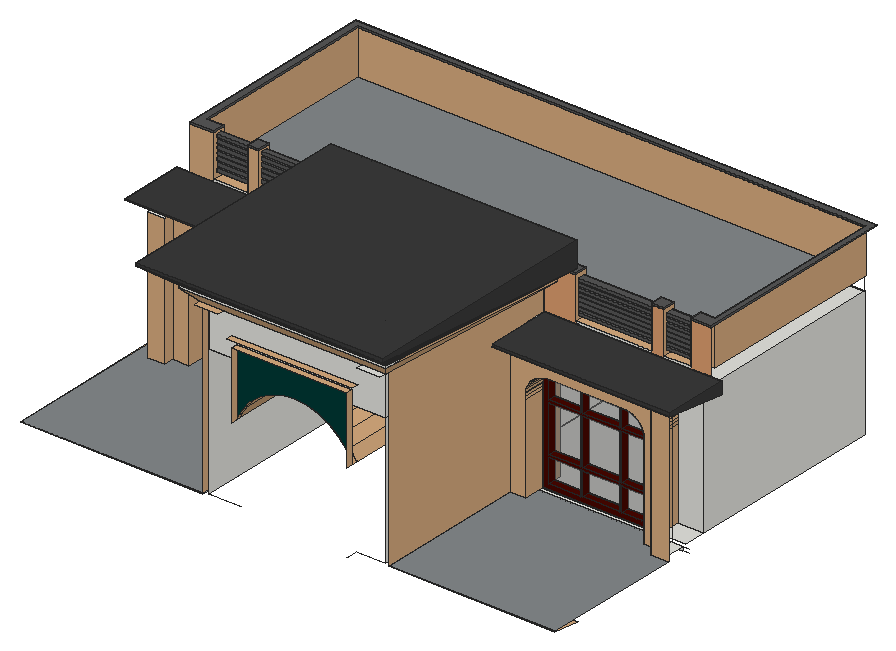
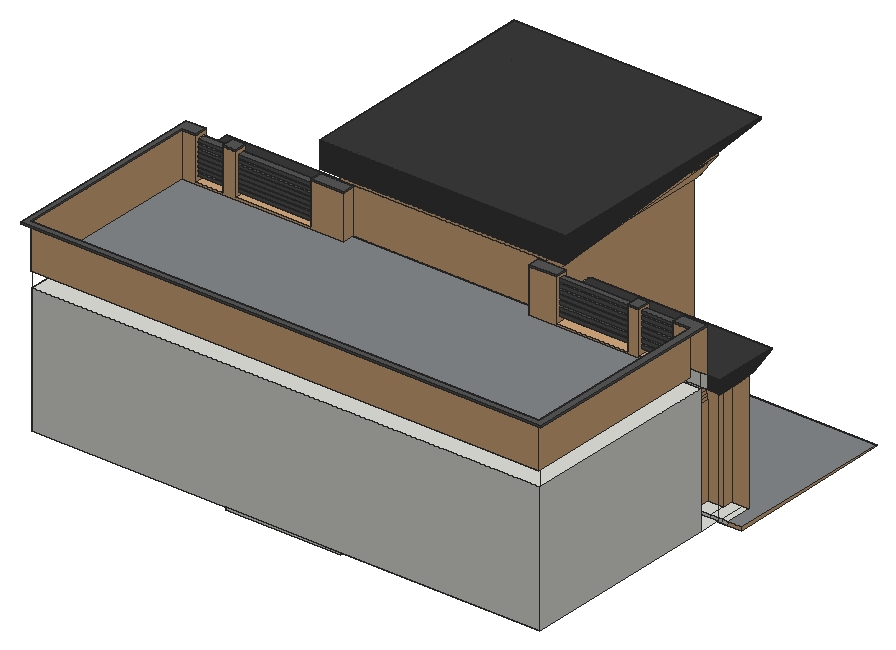
# SketchUp Ruby script. Lengths in inches.
U = 1.inch
M = Sketchup.active_model
def pt(a) = Geom::Point3d.new(a.map { |v| v * U })
def face(e, loops, mat)
  f = e.add_face(loops[0].map { |a| pt(a) })
  loops[1..].each { |l| e.add_face(l.map { |a| pt(a) }).erase! }
  f.material = f.back_material = mat if mat
  f
end
# faces: each face lists its corners as indices into pts; further lists are holes
def faces(e, pts, list, mat = nil) = list.each { |f| face(e, (f[0].is_a?(Array) ? f : [f]).map { |l| l.map { |i| pts[i] } }, mat) }
# xy, xz, yz: faces in a plane at the given z, y or x. An outline is a flat list of corners, or four numbers for a rectangle; further outlines are holes
def ring(l) = l.size == 4 ? [[l[0], l[1]], [l[2], l[1]], [l[2], l[3]], [l[0], l[3]]] : l.each_slice(2).to_a
def flat(e, list, mat, &to3) = list.each { |f| face(e, (f[0].is_a?(Array) ? f : [f]).map { |l| ring(l).map { |u, v| to3.(u, v) } }, mat) }
def xy(e, z, list, mat = nil) = flat(e, list, mat) { |x, y| [x, y, z] }
def xz(e, y, list, mat = nil) = flat(e, list, mat) { |x, z| [x, y, z] }
def yz(e, x, list, mat = nil) = flat(e, list, mat) { |y, z| [x, y, z] }
def lines(e, pts, list) = list.each { |a, b| e.add_line(pt(pts[a]), pt(pts[b])) }
# prism: a flat outline (further loops are holes) pulled along v
def prism(e, loops, v, mat = nil)
  f = face(e, loops, mat); d = Geom::Vector3d.new(v.map { |x| x * U })
  f.pushpull(f.normal.samedirection?(d) ? d.length : -d.length)
end
def box(e, o, s, mat = nil) = prism(e, [[o, [o[0] + s[0], o[1], o[2]], [o[0] + s[0], o[1] + s[1], o[2]], [o[0], o[1] + s[1], o[2]]]], [0, 0, s[2]], mat)
def at(x, y, z, deg = 0) = Geom::Transformation.translation(pt([x, y, z])) * Geom::Transformation.rotation(ORIGIN, Z_AXIS, deg.degrees)
def axes(o, x, y, z) = Geom::Transformation.new([*x, 0, *y, 0, *z, 0, *pt(o).to_a, 1])
def part(name) = M.definitions.add(name)
# library, detail: a bought-in or finely detailed component or shape, given as its bounding box
def library(name, o, s) = part(name).tap { |d| box(d.entities, o, s) }
def detail(e, o, s) = box(e.add_group.entities, o, s)
def put(e, d, t, mat = nil) = e.add_instance(d, t).tap { |i| i.material = mat if mat }
def group(e, t, mat = nil) = e.add_group.tap { |g| g.transformation = t; g.material = mat if mat }.entities
root = M.entities
M.materials.add("[Blacktop Old 01]").color = [132, 136, 139]
M.materials.add("[Checker Plate]").color = [0, 56, 52]
M.materials.add("[Color C04]").color = [215, 171, 127]
M.materials.add("[Color C04]1").color = [220, 158, 110]
M.materials.add("[Color C08]").color = [71, 7, 0]
M.materials.add("[Color M06]").color = [86, 86, 86]
M.materials.add("[Color M07]").color = [58, 58, 58]
M.materials.add("[Translucent Glass Gray]").color = [128, 128, 128]
M.materials["[Translucent Glass Gray]"].alpha = 0.5
c1 = part("Group\#1")
xy(c1.entities,0,[[0,0,133.1875,11.375]],"[Color C08]")
xy(c1.entities,6.44,[[6.44,0,42.59,11.375],[44.75,0,86.9,11.375],[89.0625,0,126.75,11.375]],"[Color C08]")
xy(c1.entities,37.85,[[6.44,0,42.59,11.375],[44.75,0,86.9,11.375],[89.0625,0,126.75,11.375]],"[Color C08]")
xy(c1.entities,40.75,[[6.44,0,42.59,11.375],[44.75,0,86.9,11.375],[89.0625,0,126.75,11.375]],"[Color C08]")
xy(c1.entities,101.6,[[6.44,0,42.59,11.375],[44.75,0,86.9,11.375],[89.0625,0,126.75,11.375]],"[Color C08]")
xy(c1.entities,104.5,[[6.44,0,42.59,11.375],[44.75,0,86.9,11.375],[89.0625,0,126.75,11.375]],"[Color C08]")
xy(c1.entities,140.62,[[24.51,0,42.59,11.375],[44.75,0,86.9,11.375],[89.0625,0,107.9,11.375]],"[Color C08]")
xy(c1.entities,147.0625,[[0,0,133.1875,11.375]],"[Color C08]")
xz(c1.entities,0,[[[0,0,133.1875,147.0625],[44.75,40.75,86.9,101.6],[89.0625,40.75,126.75,101.6],[6.44,40.75,42.59,101.6],[44.75,104.5,86.9,140.62],[44.75,6.44,86.9,37.85],[89.0625,104.5,89.0625,140.62,107.9,140.62,110.36,140.46,112.78,139.98,115.11,139.1875,117.33,138.1,119.375,136.73,121.23,135.1,122.85,133.25,124.22,131.2,125.3125,128.99,126.1,126.66,126.58,124.24,126.75,121.78,126.75,104.5],[6.44,104.5,6.44,127.03,6.65,127.83,7.8,130.52,9.36,133,11.29,135.21,13.53,137.09,16.03,138.61,18.75,139.72,21.59,140.39,24.51,140.62,42.59,140.62,42.59,104.5],[89.0625,6.44,126.75,37.85],[6.44,6.44,42.59,37.85]]],"[Color C08]")
xz(c1.entities,11.375,[[[0,0,133.1875,147.0625],[44.75,40.75,86.9,101.6],[89.0625,40.75,126.75,101.6],[6.44,40.75,42.59,101.6],[44.75,104.5,86.9,140.62],[44.75,6.44,86.9,37.85],[89.0625,104.5,126.75,104.5,126.75,121.78,126.58,124.24,126.1,126.66,125.3125,128.99,124.22,131.2,122.85,133.25,121.23,135.1,119.375,136.73,117.33,138.1,115.11,139.1875,112.78,139.98,110.36,140.46,107.9,140.62,89.0625,140.62],[6.44,104.5,42.59,104.5,42.59,140.62,24.51,140.62,21.59,140.39,18.75,139.72,16.03,138.61,13.53,137.09,11.29,135.21,9.36,133,7.8,130.52,6.65,127.83,6.44,127.03],[89.0625,6.44,126.75,37.85],[6.44,6.44,42.59,37.85]]],"[Color C08]")
xz(c1.entities,11.375,[[6.44,6.44,42.59,37.85],[44.75,6.44,86.9,37.85],[89.0625,6.44,126.75,37.85],[6.44,40.75,42.59,101.6],[44.75,40.75,86.9,101.6],
  [89.0625,40.75,126.75,101.6],[6.44,104.5,42.59,104.5,42.59,140.62,24.51,140.62,21.59,140.39,18.75,139.72,16.03,138.61,13.53,137.09,11.29,135.21,9.36,133,7.8,130.52,6.65,127.83,6.44,127.03],[44.75,104.5,86.9,140.62],[89.0625,104.5,126.75,104.5,126.75,121.78,126.58,124.24,126.1,126.66,125.3125,128.99,124.22,131.2,122.85,133.25,121.23,135.1,119.375,136.73,117.33,138.1,115.11,139.1875,112.78,139.98,110.36,140.46,107.9,140.62,89.0625,140.62]],"[Translucent Glass Gray]")
yz(c1.entities,0,[[0,0,11.375,147.0625]],"[Color C08]")
yz(c1.entities,6.44,[[0,6.44,11.375,37.85],[0,40.75,11.375,101.6],[0,104.5,11.375,127.03]],"[Color C08]")
yz(c1.entities,42.59,[[0,6.44,11.375,37.85],[0,40.75,11.375,101.6],[0,104.5,11.375,140.62]],"[Color C08]")
yz(c1.entities,44.75,[[0,6.44,11.375,37.85],[0,40.75,11.375,101.6],[0,104.5,11.375,140.62]],"[Color C08]")
yz(c1.entities,86.9,[[0,6.44,11.375,37.85],[0,40.75,11.375,101.6],[0,104.5,11.375,140.62]],"[Color C08]")
yz(c1.entities,89.0625,[[0,6.44,11.375,37.85],[0,40.75,11.375,101.6],[0,104.5,11.375,140.62]],"[Color C08]")
yz(c1.entities,126.75,[[0,6.44,11.375,37.85],[0,40.75,11.375,101.6],[0,104.5,11.375,121.78]],"[Color C08]")
yz(c1.entities,133.1875,[[0,0,11.375,147.0625]],"[Color C08]")
p = [[126.58,11.375,124.24],[126.75,11.375,121.78],[126.75,0,121.78],[126.58,0,124.24],[126.1,11.375,126.66],[126.1,0,126.66],
  [125.3125,11.375,128.99],[125.3125,0,128.99],[6.44,11.375,127.03],[6.65,11.375,127.83],[6.65,0,127.83],[6.44,0,127.03],
  [7.8,11.375,130.52],[7.8,0,130.52],[124.22,11.375,131.2],[124.22,0,131.2],[9.36,11.375,133],[9.36,0,133],
  [122.85,11.375,133.25],[122.85,0,133.25],[11.29,11.375,135.21],[11.29,0,135.21],[121.23,11.375,135.1],[121.23,0,135.1],
  [119.375,11.375,136.73],[119.375,0,136.73],[13.53,11.375,137.09],[13.53,0,137.09],[117.33,11.375,138.1],[117.33,0,138.1],
  [16.03,11.375,138.61],[16.03,0,138.61],[115.11,11.375,139.1875],[115.11,0,139.1875],[18.75,11.375,139.72],[18.75,0,139.72],
  [112.78,11.375,139.98],[112.78,0,139.98],[21.59,11.375,140.39],[21.59,0,140.39],[110.36,11.375,140.46],[110.36,0,140.46],
  [24.51,11.375,140.62],[24.51,0,140.62],[107.9,11.375,140.62],[107.9,0,140.62]]
faces(c1.entities,p,[[0,1,2,3],[4,0,3,5],[6,4,5,7],[8,9,10,11],[9,12,13,10],[14,6,7,15],[12,16,17,13],[18,14,15,19],
  [16,20,21,17],[22,18,19,23],[24,22,23,25],[20,26,27,21],[28,24,25,29],[26,30,31,27],[32,28,29,33],[30,34,35,31],
  [36,32,33,37],[34,38,39,35],[40,36,37,41],[38,42,43,39],[44,40,41,45]],"[Color C08]")
xy(root,271.1875,[[19.375,626.0625,252.9375,820.1875]])
xy(root,273.1875,[[303.29,826.22,323.73,826.22,323.73,826.24],[303.29,826.22,323.73,826.24,323.73,1134.4375,303.29,1134.4375],[323.73,826.24,323.73,1134.4375,462.79,1134.4375,462.79,826.34]])
xy(root,276.1875,[[19.375,784.25,28.375,820.1875],[28.375,784.25,42.875,820.1875],[715.65,784.25,730.375,820.1875],[42.875,798.1875,65.86,820.1875],[228.61,798.1875,252.9375,820.1875],
  [509.3125,798.1875,526.3125,820.1875],[526.3125,798.1875,531.01,820.1875],[694.01,798.1875,715.65,820.1875],[65.86,820.1875,228.61,826.1875],[531.01,820.1875,694.01,826.1875],
  [28.375,826.1875,65.86,857.1875],[65.86,826.1875,228.61,826.1875,228.61,857.1875,258.9375,857.1875,258.9375,826.1875,303.29,826.22,303.29,1134.4375,28.375,1134.4375,28.375,857.1875,65.86,857.1875],[228.61,826.1875,258.9375,857.1875],[509.3125,826.1875,509.3125,857.1875,531.01,857.1875,531.01,826.1875,694.01,826.1875,694.01,857.1875,730.375,857.1875,730.375,1134.4375,462.79,1134.4375,462.79,826.34,503.3125,826.375],[509.3125,826.1875,531.01,857.1875],
  [694.01,826.1875,730.375,857.1875],[303.29,826.22,462.79,826.34,462.79,1134.4375,303.29,1134.4375],[303.29,826.22,462.79,826.34,462.79,826.22]])
xy(root,276.1875,[[0,588.625,252.9375,588.625,252.9375,798.1875,228.61,798.1875,228.61,820.1875,65.86,820.1875,65.86,798.1875,42.875,798.1875,42.875,784.25,19.375,784.25,19.375,820.1875,0,820.1875],[509.3125,588.625,739.375,588.625,739.375,784.25,715.65,784.25,715.65,798.1875,694.01,798.1875,694.01,820.1875,531.01,820.1875,531.01,798.1875,509.3125,798.1875]],"[Blacktop Old 01]")
xy(root,428.8125,[[94.08,798.1875,199.86,857.1875]],"[Color C04]")
xy(root,434.0625,[[561.99,798.1875,665.6,857.1875]],"[Color C04]")
xy(root,454.1875,[[28.375,857.1875,730.375,1134.4375]])
xy(root,456.1875,[[258.9375,590.9375,503.3125,853.7],[715.65,784.25,715.65,798.1875,509.3125,798.1875,509.3125,857.1875,739.375,857.1875,739.375,784.25],[19.375,826.1875,19.375,857.1875,28.375,857.1875]])
xy(root,456.1875,[[739.375,784.25,739.375,857.1875,755.5,857.1875],[1.4375,826.1875,19.375,857.1875]],"[Color M07]")
xy(root,473.1875,[[509.3125,767.3125,755.5,857.1875]],"[Color M07]")
xy(root,473.8125,[[252.9375,857.1875,509.3125,857.1875,508.4375,873.75,732,873.75,732,1134.5625,29.625,1134.5625,29.625,873.75,251.9375,873.75]],"[Blacktop Old 01]")
xy(root,473.8125,[[1.4375,767.3125,252.9375,857.1875]],"[Color M07]")
xy(root,476.5625,[[52.85,857.1875,100.26,873.75],[114.72,857.1875,214.08,873.75]],"[Color C04]")
xy(root,477,[[552.94,857.1875,657.78,873.75],[674.84,857.1875,712.1,873.75]],"[Color C04]")
xy(root,480.375,[[303.29,574.1875,462.79,583.375]],"[Color C04]")
xy(root,482.68,[[548.79,860.59,712.1,870.41]],"[Color M06]")
xy(root,484.29,[[52.85,861.625,214.6,869.41]],"[Color M06]")
xy(root,486.93,[[548.79,860.59,712.1,870.41]],"[Color M06]")
xy(root,488.68,[[552.94,860.59,712.1,870.41]],"[Color M06]")
xy(root,489.0625,[[296.34,574.1875,470.03,583.375]],"[Color C04]")
xy(root,489.1,[[52.85,861.625,214.6,869.41]],"[Color M06]")
xy(root,491.35,[[52.85,861.625,219.47,869.41]],"[Color M06]")
xy(root,492.93,[[552.94,860.59,712.1,870.41]],"[Color M06]")
xy(root,494.68,[[546.92,860.59,712.1,870.41]],"[Color M06]")
xy(root,496.16,[[52.85,861.625,219.47,869.41]],"[Color M06]")
xy(root,498.41,[[52.85,861.625,218.85,869.41]],"[Color M06]")
xy(root,498.93,[[546.92,860.59,712.1,870.41]],"[Color M06]")
xy(root,500.68,[[549.67,860.59,712.1,870.41]],"[Color M06]")
xy(root,503.23,[[52.85,861.625,218.85,869.41]],"[Color M06]")
xy(root,504.93,[[549.67,860.59,712.1,870.41]],"[Color M06]")
xy(root,505.48,[[52.85,861.625,215.91,869.41]],"[Color M06]")
xy(root,506.68,[[547.98,860.59,712.1,870.41]],"[Color M06]")
xy(root,510.29,[[52.85,861.625,215.91,869.41]],"[Color M06]")
xy(root,510.93,[[547.98,860.59,712.1,870.41]],"[Color M06]")
xy(root,512.54,[[52.85,861.625,233.01,869.41]],"[Color M06]")
xy(root,512.68,[[549.67,860.59,712.1,870.41]],"[Color M06]")
xy(root,516.1875,[[477.47,573.625,509.3125,583.375]])
xy(root,516.1875,[[252.9375,573.625,285.62,583.375],[509.3125,583.375,509.3125,857.1875,526.75,857.1875]],"[Color C04]")
xy(root,516.93,[[549.67,860.59,712.1,870.41]],"[Color M06]")
xy(root,517.35,[[52.85,861.625,233.01,869.41]],"[Color M06]")
xy(root,518.68,[[549.67,860.59,712.1,870.41]],"[Color M06]")
xy(root,519.6,[[52.85,861.625,233.66,869.41]],"[Color M06]")
xy(root,522.93,[[549.67,860.59,712.1,870.41]],"[Color M06]")
xy(root,524.41,[[52.85,861.625,233.66,869.41]],"[Color M06]")
xy(root,524.68,[[541.42,860.59,712.1,870.41]],"[Color M06]")
xy(root,526.66,[[52.85,861.625,237.78,869.41]],"[Color M06]")
xy(root,528.93,[[541.42,860.59,712.1,870.41]],"[Color M06]")
xy(root,531.48,[[52.85,861.625,237.78,869.41]],"[Color M06]")
xy(root,533.8125,[[19.375,857.1875,19.375,1143.4375,739.375,1143.4375,739.375,857.1875,712.1,857.1875,712.1,873.75,732,873.75,732,1134.5625,29.625,1134.5625,29.625,873.75,52.85,873.75,52.85,857.1875],[100.26,857.1875,114.72,873.75],[214.08,857.1875,214.08,873.75,251.9375,873.75,252.9375,857.1875],[509.3125,857.1875,508.4375,873.75,552.94,873.75,552.94,857.1875],[657.78,857.1875,674.84,873.75]])
xy(root,536.25,[[19.375,857.1875,52.85,857.1875,52.85,873.75,29.625,873.75,29.625,1134.5625,732,1134.5625,732,873.75,712.1,873.75,712.1,857.1875,739.375,857.1875,739.375,1143.4375,19.375,1143.4375],[100.26,857.1875,114.72,873.75],[214.08,857.1875,252.9375,857.1875,251.9375,873.75,214.08,873.75],[509.3125,857.1875,552.94,857.1875,552.94,873.75,508.4375,873.75],[657.78,857.1875,674.84,873.75]],"[Color M06]")
xy(root,537.625,[[[240.4375,561.625,526.75,857.1875],[258.9375,590.9375,503.3125,853.7]],[258.9375,590.9375,503.3125,853.7]])
xy(root,541.625,[[[240.4375,561.625,526.75,857.1875],[258.9375,590.9375,503.3125,853.7]]])
xy(root,541.625,[[526.75,561.625,526.75,857.1875,554.625,857.1875]],"[Color M07]")
xy(root,577.625,[[213.875,521,554.625,857.1875]],"[Color M07]")
xz(root,521,[[213.875,573.66,554.625,577.625]],"[Color M07]")
xz(root,561.625,[[240.4375,537.625,526.75,541.625]])
xz(root,583.375,[[303.29,387.35,311.2,402.37,321.89,415.55,334.97,426.37,349.92,434.41,366.15,439.37,383.04,441.04,399.93,439.37,416.16,434.41,431.11,426.37,444.18,415.55,454.88,402.37,462.79,387.35,462.79,480.375,303.29,480.375]],"[Checker Plate]")
xz(root,588.625,[[0,275.59,252.9375,276.1875],[509.3125,275.59,739.375,276.1875]])
xz(root,590.9375,[[258.9375,456.1875,503.3125,516.1875],[258.9375,516.1875,503.3125,537.625],[258.9375,537.625,503.3125,541.625]])
xz(root,767.3125,[[509.3125,468.6,755.5,473.1875],[1.4375,472.11,252.9375,473.8125]],"[Color M07]")
xz(root,784.25,[[19.375,276.1875,42.875,456.1875],[715.65,276.1875,739.375,456.1875]],"[Color C04]")
xz(root,798.1875,[[42.875,276.1875,65.86,276.1875,65.86,400.6,66.1,404.28,66.82,407.9,68.01,411.39,69.64,414.7,71.69,417.77,74.125,420.55,76.9,422.98,79.97,425.03,83.28,426.66,86.77,427.85,90.39,428.57,94.08,428.8125,199.86,428.8125,203.61,428.57,207.3,427.83,210.86,426.625,214.23,424.96,217.36,422.87,220.1875,420.39,222.67,417.5625,224.76,414.4375,226.42,411.0625,227.63,407.5,228.36,403.8125,228.61,400.06,228.61,276.1875,252.9375,276.1875,252.9375,458.3,42.875,458.3],[509.3125,276.1875,531.01,276.1875,531.01,397.35,530.58,401.89,530.8,406.43,531.01,407.55,531.67,410.9,533.18,415.19,535.3,419.22,537.97,422.9,541.15,426.16,544.77,428.92,548.75,431.14,553,432.75,557.45,433.73,561.99,434.0625,665.6,434.0625,669.93,433.74,674.17,432.77,678.22,431.1875,681.98,429.02,685.38,426.3125,688.34,423.13,690.8,419.55,692.6875,415.64,693.98,411.49,694.01,411.25,694.64,407.19,694.65,402.85,694.01,398.55,694.01,276.1875,715.65,276.1875,715.65,456.1875,509.3125,456.1875]],"[Color C04]")
xz(root,820.1875,[[19.375,271.1875,28.375,276.1875],[28.375,271.1875,42.875,276.1875],[42.875,271.1875,252.9375,276.1875],[509.3125,271.1875,526.3125,276.1875],[526.3125,271.1875,730.375,276.1875]])
xz(root,820.1875,[[0,271.1875,19.375,276.1875]],"[Color C04]")
xz(root,826.22,[[303.29,273.1875,323.73,276.1875],[303.29,276.1875,462.79,276.1875,462.79,387.35,454.88,402.37,444.18,415.55,431.11,426.37,416.16,434.41,399.93,439.37,383.04,441.04,366.15,439.37,349.92,434.41,334.97,426.37,321.89,415.55,311.2,402.37,303.29,387.35]])
xz(root,853.7,[[258.9375,456.1875,503.3125,516.1875],[258.9375,516.1875,503.3125,537.625],[258.9375,537.625,273,541.625],[273,537.625,503.3125,541.625]])
xz(root,857.1875,[[28.375,276.1875,28.375,454.1875,258.9375,454.1875,258.9375,276.1875,228.61,276.1875,228.61,400.06,228.36,403.8125,227.63,407.5,226.42,411.0625,224.76,414.4375,222.67,417.5625,220.1875,420.39,217.36,422.87,214.23,424.96,210.86,426.625,207.3,427.83,203.61,428.57,199.86,428.8125,94.08,428.8125,90.39,428.57,86.77,427.85,83.28,426.66,79.97,425.03,76.9,422.98,74.125,420.55,71.69,417.77,69.64,414.7,68.01,411.39,66.82,407.9,66.1,404.28,65.86,400.6,65.86,276.1875],[509.3125,276.1875,509.3125,454.1875,730.375,454.1875,730.375,276.1875,694.01,276.1875,694.01,398.55,694.65,402.85,694.64,407.19,694.01,411.25,693.98,411.49,692.6875,415.64,690.8,419.55,688.34,423.13,685.38,426.3125,681.98,429.02,678.22,431.1875,674.17,432.77,669.93,433.74,665.6,434.0625,561.99,434.0625,557.45,433.73,553,432.75,548.75,431.14,544.77,428.92,541.15,426.16,537.97,422.9,535.3,419.22,533.18,415.19,531.67,410.9,531.01,407.55,530.8,406.43,530.58,401.89,531.01,397.35,531.01,276.1875],[28.375,454.1875,252.9375,456.1875],[252.9375,454.1875,258.9375,473.8125],[258.9375,454.1875,509.3125,473.8125],
  [509.3125,454.1875,730.375,456.1875],[19.375,456.1875,28.375,473.8125],[28.375,456.1875,252.9375,473.8125],[509.3125,456.1875,730.375,473.1875],[730.375,456.1875,739.375,473.1875],
  [509.3125,473.1875,552.94,473.8125],[552.94,473.1875,730.375,473.8125],[730.375,473.1875,739.375,473.8125],[52.85,473.8125,100.26,476.5625],[114.72,473.8125,214.08,476.5625],
  [552.94,473.8125,657.78,477],[674.84,473.8125,712.1,477],[240.4375,516.1875,252.9375,533.8125],[509.3125,516.1875,526.75,533.8125],[240.4375,533.8125,252.9375,536.25],
  [509.3125,533.8125,526.75,536.25]])
xz(root,857.1875,[[19.375,473.8125,52.85,533.8125],[100.26,473.8125,114.72,533.8125],[214.08,473.8125,252.9375,473.8125,252.9375,516.1875,240.4375,516.1875,240.4375,533.8125,214.08,533.8125],[252.9375,473.8125,252.9375,536.25,240.4375,536.25,240.4375,537.625,526.75,537.625,526.75,536.25,509.3125,536.25,509.3125,473.8125],[240.4375,537.625,526.75,541.625]],"[Color C04]")
xz(root,857.1875,[[509.3125,473.8125,552.94,473.8125,552.94,533.8125,526.75,533.8125,526.75,516.1875,509.3125,516.1875],[657.78,473.8125,674.84,533.8125],[712.1,473.8125,739.375,533.8125]],"[Color C04]1")
xz(root,857.1875,[[19.375,533.8125,52.85,536.25],[100.26,533.8125,114.72,536.25],[214.08,533.8125,240.4375,536.25],[526.75,533.8125,552.94,536.25],[657.78,533.8125,674.84,536.25],
  [712.1,533.8125,739.375,536.25]],"[Color M06]")
xz(root,857.1875,[[1.4375,456.1875,19.375,473.8125],[739.375,456.1875,755.5,473.1875],[213.875,541.625,554.625,577.625]],"[Color M07]")
xz(root,860.59,[[548.79,482.68,712.1,486.93],[552.94,488.68,712.1,492.93],[546.92,494.68,712.1,498.93],[549.67,500.68,712.1,504.93],[547.98,506.68,712.1,510.93],
  [549.67,512.68,712.1,516.93],[549.67,518.68,712.1,522.93],[541.42,524.68,712.1,528.93]],"[Color M06]")
xz(root,861.625,[[52.85,484.29,214.6,489.1],[52.85,491.35,219.47,496.16],[52.85,498.41,218.85,503.23],[52.85,505.48,215.91,510.29],[52.85,512.54,233.01,517.35],
  [52.85,519.6,233.66,524.41],[52.85,526.66,237.78,531.48]],"[Color M06]")
xz(root,869.41,[[52.85,484.29,214.6,489.1],[52.85,491.35,219.47,496.16],[52.85,498.41,218.85,503.23],[52.85,505.48,215.91,510.29],[52.85,512.54,233.01,517.35],
  [52.85,519.6,233.66,524.41],[52.85,526.66,237.78,531.48]],"[Color M06]")
xz(root,870.41,[[548.79,482.68,712.1,486.93],[552.94,488.68,712.1,492.93],[546.92,494.68,712.1,498.93],[549.67,500.68,712.1,504.93],[547.98,506.68,712.1,510.93],
  [549.67,512.68,712.1,516.93],[549.67,518.68,712.1,522.93],[541.42,524.68,712.1,528.93]],"[Color M06]")
xz(root,873.75,[[29.625,473.8125,29.625,533.8125,52.85,533.8125,52.85,476.5625,100.26,476.5625,100.26,533.8125,114.72,533.8125,114.72,476.5625,214.08,476.5625,214.08,533.8125,251.9375,533.8125,251.9375,473.8125],[508.4375,473.8125,508.4375,533.8125,552.94,533.8125,552.94,477,657.78,477,657.78,533.8125,674.84,533.8125,674.84,477,712.1,477,712.1,533.8125,732,533.8125,732,473.8125]],"[Color C04]")
xz(root,873.75,[[29.625,533.8125,52.85,536.25],[100.26,533.8125,114.72,536.25],[214.08,533.8125,251.9375,536.25],[508.4375,533.8125,552.94,536.25],[657.78,533.8125,674.84,536.25],
  [712.1,533.8125,732,536.25]],"[Color M06]")
xz(root,1134.4375,[[303.29,273.1875,462.79,276.1875],[28.375,276.1875,730.375,454.1875]])
xz(root,1134.5625,[[29.625,473.8125,732,533.8125]],"[Color C04]")
xz(root,1134.5625,[[29.625,533.8125,732,536.25]],"[Color M06]")
xz(root,1143.4375,[[19.375,533.8125,739.375,536.25]],"[Color M06]")
yz(root,0,[[820.1875,271.1875,588.625,275.59,588.625,276.1875,820.1875,276.1875]],"[Color C04]")
yz(root,1.4375,[[826.1875,456.1875,798.1875,458.3,767.3125,472.11,767.3125,473.8125,857.1875,473.8125,857.1875,456.1875]],"[Color M07]")
yz(root,19.375,[[857.1875,533.8125,1143.4375,536.25]],"[Color M06]")
yz(root,28.375,[[857.1875,276.1875,1134.4375,454.1875]])
yz(root,29.625,[[873.75,473.8125,1134.5625,533.8125]],"[Color C04]")
yz(root,29.625,[[873.75,533.8125,1134.5625,536.25]],"[Color M06]")
yz(root,42.875,[[784.25,276.1875,798.1875,276.1875,798.1875,458.3,784.25,456.1875]],"[Color C04]")
yz(root,52.85,[[861.625,484.29,869.41,489.1],[861.625,491.35,869.41,496.16],[861.625,498.41,869.41,503.23],[861.625,505.48,869.41,510.29],[861.625,512.54,869.41,517.35],
  [861.625,519.6,869.41,524.41],[861.625,526.66,869.41,531.48]])
yz(root,52.85,[[[857.1875,476.5625,873.75,533.8125],[861.625,526.66,869.41,531.48],[861.625,519.6,869.41,524.41],[861.625,512.54,869.41,517.35],[861.625,505.48,869.41,510.29],[861.625,498.41,869.41,503.23],[861.625,491.35,869.41,496.16],[861.625,484.29,869.41,489.1]]],"[Color C04]")
yz(root,52.85,[[857.1875,533.8125,873.75,536.25]],"[Color M06]")
yz(root,65.86,[[798.1875,276.1875,857.1875,400.6]],"[Color C04]")
yz(root,100.26,[[857.1875,476.5625,873.75,533.8125]],"[Color C04]")
yz(root,100.26,[[857.1875,533.8125,873.75,536.25]],"[Color M06]")
yz(root,114.72,[[857.1875,476.5625,873.75,533.8125]],"[Color C04]")
yz(root,114.72,[[857.1875,533.8125,873.75,536.25]],"[Color M06]")
yz(root,213.875,[[857.1875,541.625,521,573.66,521,577.625,857.1875,577.625]],"[Color M07]")
yz(root,214.08,[[857.1875,476.5625,873.75,533.8125]],"[Color C04]")
yz(root,214.08,[[857.1875,533.8125,873.75,536.25]],"[Color M06]")
yz(root,214.6,[[861.625,484.29,869.41,489.1]])
yz(root,215.91,[[861.625,505.48,869.41,510.29]])
yz(root,218.85,[[861.625,498.41,869.41,503.23]])
yz(root,219.47,[[861.625,491.35,869.41,496.16]])
yz(root,228.61,[[798.1875,276.1875,857.1875,400.06]],"[Color C04]")
yz(root,233.01,[[861.625,512.54,869.41,517.35]])
yz(root,233.66,[[861.625,519.6,869.41,524.41]])
yz(root,237.78,[[861.625,526.66,869.41,531.48]])
yz(root,240.4375,[[857.1875,516.1875,561.625,537.625,857.1875,537.625],[561.625,537.625,857.1875,541.625]],"[Color C04]")
yz(root,252.9375,[[626.0625,271.1875,626.0625,276.1875,588.625,276.1875,588.625,275.59],[626.0625,271.1875,638.0625,276.1875],[638.0625,271.1875,820.1875,276.1875],[857.1875,456.1875,798.1875,458.3,767.3125,472.11,767.3125,473.8125,857.1875,473.8125]])
yz(root,252.9375,[[588.625,276.1875,588.625,516.1875,857.1875,516.1875,857.1875,473.8125,767.3125,473.8125,767.3125,472.11,798.1875,458.3,798.1875,276.1875]],"[Color C04]")
yz(root,258.9375,[[590.9375,276.1875,857.1875,456.1875],[590.9375,456.1875,853.7,516.1875],[590.9375,516.1875,853.7,537.625],[590.9375,537.625,853.7,541.625]])
yz(root,303.29,[[826.22,273.1875,1134.4375,276.1875]])
yz(root,303.29,[[574.1875,387.35,583.375,480.375]],"[Color C04]")
yz(root,462.79,[[826.34,273.1875,1134.4375,276.1875]])
yz(root,462.79,[[574.1875,387.35,583.375,480.375]],"[Color C04]")
yz(root,503.3125,[[590.9375,276.1875,826.375,456.1875],[590.9375,456.1875,853.7,516.1875],[590.9375,516.1875,853.7,537.625],[590.9375,537.625,853.7,541.625]])
yz(root,509.3125,[[627.4375,271.1875,588.625,275.59,588.625,276.1875,627.4375,276.1875],[627.4375,271.1875,638.0625,276.1875],[638.0625,271.1875,820.1875,276.1875],[826.1875,276.1875,857.1875,456.1875],[798.1875,456.1875,826.1875,456.1875,826.1875,473.1875,767.3125,473.1875,767.3125,468.6],
  [826.1875,456.1875,857.1875,473.1875]])
yz(root,509.3125,[[588.625,276.1875,798.1875,276.1875,798.1875,456.1875,767.3125,468.6,767.3125,473.1875,857.1875,473.1875,857.1875,516.1875,588.625,516.1875]],"[Color C04]")
yz(root,526.75,[[561.625,537.625,857.1875,541.625]])
yz(root,526.75,[[857.1875,516.1875,857.1875,537.625,561.625,537.625]],"[Color C04]")
yz(root,531.01,[[798.1875,276.1875,857.1875,397.35]],"[Color C04]")
yz(root,541.42,[[860.59,524.68,870.41,528.93]])
yz(root,546.92,[[860.59,494.68,870.41,498.93]])
yz(root,547.98,[[860.59,506.68,870.41,510.93]])
yz(root,548.79,[[860.59,482.68,870.41,486.93]])
yz(root,549.67,[[860.59,500.68,870.41,504.93],[860.59,512.68,870.41,516.93],[860.59,518.68,870.41,522.93]])
yz(root,552.94,[[[857.1875,477,873.75,533.8125],[860.59,488.68,870.41,492.93]]],"[Color C04]")
yz(root,552.94,[[857.1875,533.8125,873.75,536.25]],"[Color M06]")
yz(root,554.625,[[857.1875,541.625,857.1875,577.625,521,577.625,521,573.66]],"[Color M07]")
yz(root,657.78,[[857.1875,477,873.75,533.8125]],"[Color C04]")
yz(root,657.78,[[857.1875,533.8125,873.75,536.25]],"[Color M06]")
yz(root,674.84,[[857.1875,477,873.75,533.8125]],"[Color C04]")
yz(root,674.84,[[857.1875,533.8125,873.75,536.25]],"[Color M06]")
yz(root,694.01,[[798.1875,276.1875,857.1875,398.55]],"[Color C04]")
yz(root,712.1,[[860.59,482.68,870.41,486.93],[860.59,488.68,870.41,492.93],[860.59,494.68,870.41,498.93],[860.59,500.68,870.41,504.93],[860.59,506.68,870.41,510.93],
  [860.59,512.68,870.41,516.93],[860.59,518.68,870.41,522.93],[860.59,524.68,870.41,528.93]])
yz(root,712.1,[[[857.1875,477,873.75,533.8125],[860.59,482.68,870.41,486.93],[860.59,488.68,870.41,492.93],[860.59,494.68,870.41,498.93],[860.59,500.68,870.41,504.93],[860.59,506.68,870.41,510.93],[860.59,512.68,870.41,516.93],[860.59,518.68,870.41,522.93],[860.59,524.68,870.41,528.93]]],"[Color C04]")
yz(root,712.1,[[857.1875,533.8125,873.75,536.25]],"[Color M06]")
yz(root,715.65,[[784.25,276.1875,798.1875,456.1875]],"[Color C04]")
yz(root,730.375,[[857.1875,276.1875,1134.4375,454.1875]])
yz(root,732,[[873.75,473.8125,1134.5625,533.8125]],"[Color C04]")
yz(root,732,[[873.75,533.8125,1134.5625,536.25]],"[Color M06]")
yz(root,739.375,[[857.1875,533.8125,1143.4375,536.25]],"[Color M06]")
yz(root,755.5,[[857.1875,456.1875,857.1875,473.1875,767.3125,473.1875,767.3125,468.6]],"[Color M07]")
p = [[0,820.1875,271.1875],[19.375,820.1875,271.1875],[0,588.625,275.59],[19.375,626.0625,271.1875],[252.9375,626.0625,271.1875],[252.9375,588.625,275.59],
  [509.3125,627.4375,271.1875],[739.375,627.4375,271.1875],[739.375,588.625,275.59],[509.3125,588.625,275.59],[462.79,826.34,276.1875],[303.29,826.22,276.1875],
  [303.29,826.22,273.1875],[323.73,826.24,273.1875],[462.79,826.34,273.1875],[311.2,583.375,402.37],[303.29,583.375,387.35],[303.29,590.9375,387.35],
  [311.2,590.9375,402.37],[462.79,583.375,387.35],[454.88,583.375,402.37],[454.88,590.9375,402.37],[462.79,590.9375,387.35],[311.2,826.22,402.37],
  [303.29,826.22,387.35],[462.79,826.22,387.35],[454.88,826.22,402.37],[530.58,857.1875,401.89],[530.58,798.1875,401.89],[531.01,798.1875,397.35],
  [531.01,857.1875,397.35],[694.01,857.1875,398.55],[694.01,798.1875,398.55],[694.65,798.1875,402.85],[694.65,857.1875,402.85],[228.61,857.1875,400.06],
  [228.61,798.1875,400.06],[228.36,798.1875,403.8125],[228.36,857.1875,403.8125],[66.1,857.1875,404.28],[66.1,798.1875,404.28],[65.86,798.1875,400.6],
  [65.86,857.1875,400.6],[530.8,857.1875,406.43],[530.8,798.1875,406.43],[321.89,583.375,415.55],[321.89,590.9375,415.55],[444.18,583.375,415.55],
  [444.18,590.9375,415.55],[321.89,826.22,415.55],[444.18,826.22,415.55],[694.64,798.1875,407.19],[694.64,857.1875,407.19],[227.63,798.1875,407.5],
  [227.63,857.1875,407.5],[66.82,857.1875,407.9],[66.82,798.1875,407.9],[531.01,857.1875,407.55],[531.01,798.1875,407.55],[694.01,798.1875,411.25],
  [694.01,857.1875,411.25],[226.42,798.1875,411.0625],[226.42,857.1875,411.0625],[531.67,857.1875,410.9],[531.67,798.1875,410.9],[68.01,857.1875,411.39],
  [68.01,798.1875,411.39],[533.18,857.1875,415.19],[533.18,798.1875,415.19],[224.76,798.1875,414.4375],[224.76,857.1875,414.4375],[693.98,798.1875,411.49],
  [693.98,857.1875,411.49],[69.64,857.1875,414.7],[69.64,798.1875,414.7],[692.6875,798.1875,415.64],[692.6875,857.1875,415.64],[222.67,798.1875,417.5625],
  [222.67,857.1875,417.5625],[71.69,857.1875,417.77],[71.69,798.1875,417.77],[535.3,857.1875,419.22],[535.3,798.1875,419.22],[334.97,583.375,426.37],
  [334.97,590.9375,426.37],[431.11,583.375,426.37],[431.11,590.9375,426.37],[334.97,826.22,426.37],[431.11,826.22,426.37],[690.8,798.1875,419.55],
  [690.8,857.1875,419.55],[220.1875,798.1875,420.39],[220.1875,857.1875,420.39],[74.125,857.1875,420.55],[74.125,798.1875,420.55],[537.97,857.1875,422.9],
  [537.97,798.1875,422.9],[688.34,798.1875,423.13],[688.34,857.1875,423.13],[217.36,798.1875,422.87],[217.36,857.1875,422.87],[76.9,857.1875,422.98],
  [76.9,798.1875,422.98],[214.23,798.1875,424.96],[214.23,857.1875,424.96],[541.15,857.1875,426.16],[541.15,798.1875,426.16],[79.97,857.1875,425.03],
  [79.97,798.1875,425.03],[685.38,798.1875,426.3125],[685.38,857.1875,426.3125],[83.28,857.1875,426.66],[83.28,798.1875,426.66],[210.86,798.1875,426.625],
  [210.86,857.1875,426.625],[544.77,857.1875,428.92],[544.77,798.1875,428.92],[681.98,798.1875,429.02],[681.98,857.1875,429.02],[349.92,583.375,434.41],
  [349.92,590.9375,434.41],[416.16,583.375,434.41],[416.16,590.9375,434.41],[349.92,826.22,434.41],[416.16,826.22,434.41],[207.3,798.1875,427.83],
  [207.3,857.1875,427.83],[86.77,857.1875,427.85],[86.77,798.1875,427.85],[203.61,798.1875,428.57],[203.61,857.1875,428.57],[90.39,857.1875,428.57],
  [90.39,798.1875,428.57],[94.08,857.1875,428.8125],[94.08,798.1875,428.8125],[199.86,798.1875,428.8125],[199.86,857.1875,428.8125],[548.75,857.1875,431.14],
  [548.75,798.1875,431.14],[678.22,798.1875,431.1875],[678.22,857.1875,431.1875],[553,857.1875,432.75],[553,798.1875,432.75],[674.17,798.1875,432.77],
  [674.17,857.1875,432.77],[557.45,857.1875,433.73],[557.45,798.1875,433.73],[669.93,798.1875,433.74],[669.93,857.1875,433.74],[561.99,857.1875,434.0625],
  [561.99,798.1875,434.0625],[665.6,798.1875,434.0625],[665.6,857.1875,434.0625],[366.15,583.375,439.37],[366.15,590.9375,439.37],[399.93,583.375,439.37],
  [399.93,590.9375,439.37],[366.15,826.22,439.37],[399.93,826.22,439.37],[383.04,583.375,441.04],[383.04,590.9375,441.04],[383.04,826.22,441.04],
  [509.3125,798.1875,456.1875],[715.65,798.1875,456.1875],[509.3125,767.3125,468.6],[715.65,784.25,456.1875],[739.375,784.25,456.1875],[755.5,767.3125,468.6],
  [755.5,857.1875,456.1875],[19.375,784.25,456.1875],[42.875,784.25,456.1875],[42.875,798.1875,458.3],[19.375,798.1875,458.3],[19.375,826.1875,456.1875],
  [1.4375,798.1875,458.3],[1.4375,826.1875,456.1875],[28.375,857.1875,456.1875],[252.9375,857.1875,456.1875],[252.9375,798.1875,458.3],[252.9375,767.3125,472.11],
  [1.4375,767.3125,472.11],[252.9375,857.1875,473.8125],[251.9375,873.75,473.8125],[251.9375,873.75,533.8125],[252.9375,857.1875,533.8125],[252.9375,857.1875,516.1875],
  [508.4375,873.75,473.8125],[509.3125,857.1875,473.8125],[509.3125,857.1875,516.1875],[509.3125,857.1875,533.8125],[508.4375,873.75,533.8125],[240.4375,857.1875,516.1875],
  [240.4375,561.625,537.625],[252.9375,588.625,516.1875],[252.9375,583.375,516.1875],[285.62,583.375,516.1875],[477.47,583.375,516.1875],[509.3125,583.375,516.1875],
  [526.75,561.625,537.625],[526.75,857.1875,516.1875],[251.9375,873.75,536.25],[252.9375,857.1875,536.25],[509.3125,857.1875,536.25],[508.4375,873.75,536.25],
  [240.4375,561.625,541.625],[213.875,521,573.66],[240.4375,857.1875,541.625],[526.75,561.625,541.625],[554.625,521,573.66],[213.875,857.1875,541.625],
  [554.625,857.1875,541.625],[739.375,820.1875,271.1875],[730.375,820.1875,271.1875],[739.375,820.1875,276.1875],[730.375,820.1875,276.1875],[258.9375,590.9375,276.1875],
  [303.29,590.9375,276.1875],[28.375,826.1875,276.1875],[28.375,826.1875,456.1875],[715.65,820.1875,456.1875],[715.65,820.1875,276.1875],[503.3125,853.7,541.625],
  [503.3125,853.7,577.625],[273,853.7,541.625],[273,853.7,577.625],[503.3125,590.9375,541.625],[503.3125,590.9375,577.625],[258.9375,853.7,541.625],
  [258.9375,853.7,577.625],[462.79,590.9375,276.1875],[503.3125,590.9375,276.1875],[462.79,574.1875,276.1875],[730.375,1134.4375,454.1875],[730.375,1134.4375,473.8125],
  [28.375,1134.4375,454.1875],[28.375,1134.4375,473.8125]]
faces(root,p,[[0,1,2],[3,2,1],[2,3,4,5],[6,7,8,9],[15,16,17,18],[19,20,21,22],[23,18,17,24],[25,22,21,26],
  [27,28,29,30],[31,32,33,34],[35,36,37,38],[39,40,41,42],[43,44,28,27],[45,15,18,46],[20,47,48,21],[49,46,18,23],
  [26,21,48,50],[34,33,51,52],[38,37,53,54],[55,56,40,39],[57,58,44,43],[52,51,59,60],[54,53,61,62],[63,64,58,57],
  [65,66,56,55],[67,68,64,63],[62,61,69,70],[60,59,71,72],[73,74,66,65],[72,71,75,76],[70,69,77,78],[79,80,74,73],
  [81,82,68,67],[83,45,46,84],[47,85,86,48],[87,84,46,49],[50,48,86,88],[76,75,89,90],[78,77,91,92],[93,94,80,79],
  [95,96,82,81],[90,89,97,98],[92,91,99,100],[101,102,94,93],[100,99,103,104],[105,106,96,95],[107,108,102,101],[98,97,109,110],
  [111,112,108,107],[104,103,113,114],[115,116,106,105],[110,109,117,118],[119,83,84,120],[85,121,122,86],[123,120,84,87],[88,86,122,124],
  [114,113,125,126],[127,128,112,111],[126,125,129,130],[131,132,128,127],[133,134,132,131],[130,129,135,136],[137,138,116,115],[118,117,139,140],
  [141,142,138,137],[140,139,143,144],[145,146,142,141],[144,143,147,148],[149,150,146,145],[148,147,151,152],[153,119,120,154],[121,155,156,122],
  [157,154,120,123],[124,122,156,158],[159,153,154,160],[155,159,160,156],[161,160,154,157],[158,156,160,161],[181,182,183,184,185],[186,187,188,189,190],
  [191,185,192],[192,185,193,194],[192,194,195,196,197,198],[199,198,197]],"[Color C04]")
faces(root,p,[[10,11,12,13,14],[169,170,171,172],[172,173,176],[176,177,178,171,172]])
faces(root,p,[[162,163,164],[165,164,163],[164,165,166,167],[168,167,166],[173,172,174,175],[172,171,178,179,180,174],[204,205,206],[205,204,207,208],
  [209,206,205],[210,208,207]],"[Color M07]")
faces(root,p,[[184,183,200,201],[190,189,202,203]],"[Color M06]")
lines(root,p,[[211,212],[213,214],[215,216],[217,218],[219,220],[221,222],[223,224],[225,226],[227,228],[229,230],[229,231],[232,233],
  [234,235]])
put(root,c1,axes([68.78,826.1875,276.1875],[1.2,0,0],[0,1,0],[0,0,1.03782]))
put(root,c1,axes([531.01,827.75,276.1875],[1.22384,0,0],[0,1,0],[0,0,1.05858]))
